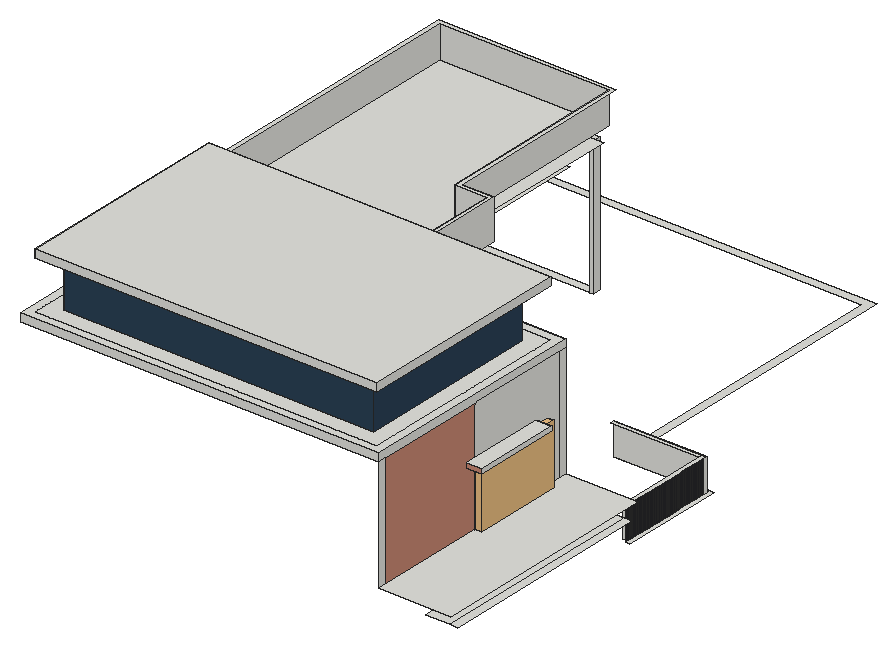
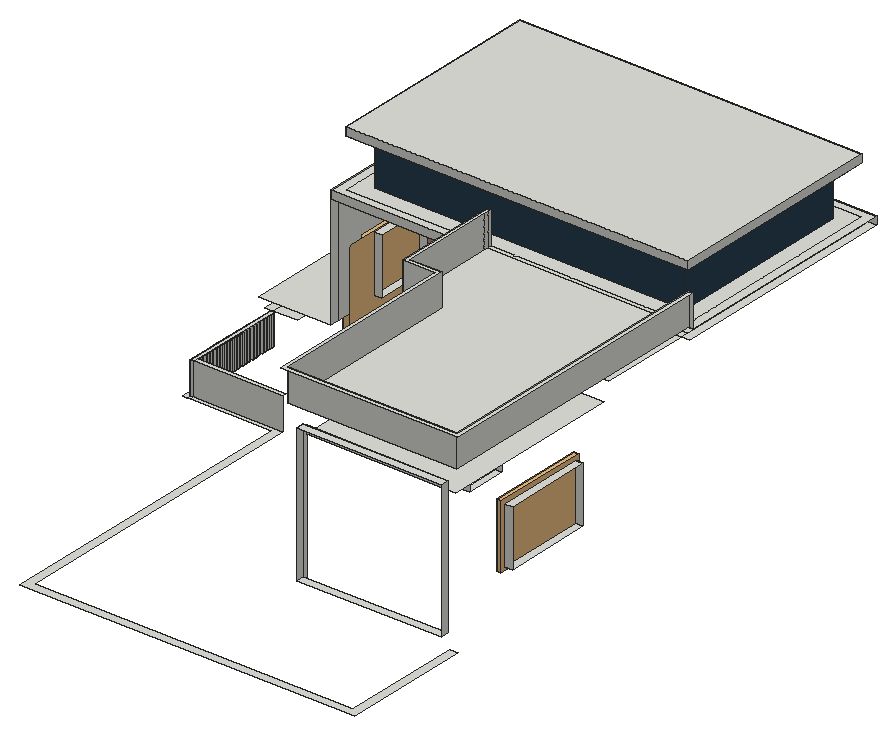
# SketchUp Ruby script. Lengths in inches.
U = 1.inch
M = Sketchup.active_model
def pt(a) = Geom::Point3d.new(a.map { |v| v * U })
def face(e, loops, mat)
  f = e.add_face(loops[0].map { |a| pt(a) })
  loops[1..].each { |l| e.add_face(l.map { |a| pt(a) }).erase! }
  f.material = f.back_material = mat if mat
  f
end
# faces: each face lists its corners as indices into pts; further lists are holes
def faces(e, pts, list, mat = nil) = list.each { |f| face(e, (f[0].is_a?(Array) ? f : [f]).map { |l| l.map { |i| pts[i] } }, mat) }
# xy, xz, yz: faces in a plane at the given z, y or x. An outline is a flat list of corners, or four numbers for a rectangle; further outlines are holes
def ring(l) = l.size == 4 ? [[l[0], l[1]], [l[2], l[1]], [l[2], l[3]], [l[0], l[3]]] : l.each_slice(2).to_a
def flat(e, list, mat, &to3) = list.each { |f| face(e, (f[0].is_a?(Array) ? f : [f]).map { |l| ring(l).map { |u, v| to3.(u, v) } }, mat) }
def xy(e, z, list, mat = nil) = flat(e, list, mat) { |x, y| [x, y, z] }
def xz(e, y, list, mat = nil) = flat(e, list, mat) { |x, z| [x, y, z] }
def yz(e, x, list, mat = nil) = flat(e, list, mat) { |y, z| [x, y, z] }
def lines(e, pts, list) = list.each { |a, b| e.add_line(pt(pts[a]), pt(pts[b])) }
# prism: a flat outline (further loops are holes) pulled along v
def prism(e, loops, v, mat = nil)
  f = face(e, loops, mat); d = Geom::Vector3d.new(v.map { |x| x * U })
  f.pushpull(f.normal.samedirection?(d) ? d.length : -d.length)
end
def box(e, o, s, mat = nil) = prism(e, [[o, [o[0] + s[0], o[1], o[2]], [o[0] + s[0], o[1] + s[1], o[2]], [o[0], o[1] + s[1], o[2]]]], [0, 0, s[2]], mat)
def at(x, y, z, deg = 0) = Geom::Transformation.translation(pt([x, y, z])) * Geom::Transformation.rotation(ORIGIN, Z_AXIS, deg.degrees)
def axes(o, x, y, z) = Geom::Transformation.new([*x, 0, *y, 0, *z, 0, *pt(o).to_a, 1])
def part(name) = M.definitions.add(name)
# library, detail: a bought-in or finely detailed component or shape, given as its bounding box
def library(name, o, s) = part(name).tap { |d| box(d.entities, o, s) }
def detail(e, o, s) = box(e.add_group.entities, o, s)
def put(e, d, t, mat = nil) = e.add_instance(d, t).tap { |i| i.material = mat if mat }
def group(e, t, mat = nil) = e.add_group.tap { |g| g.transformation = t; g.material = mat if mat }.entities
root = M.entities
M.materials.add("Brick_10_1K").color = [200, 136, 115]
M.materials.add("Carpet_04_1K").color = [43, 65, 85]
M.materials.add("ThomThom - Buttons2").color = [40, 40, 43]
c1 = library("mesh-162",[-1607.75,-1245.64,-53.98],[1739.16,1702.88,120.91])
c2 = part("Group9\#1")
put(c2.entities,c1,at(0,0,0))
xy(root,129,[[162,247.5,166.5,277.5]])
xy(root,132,[[357,219,360,297],[288,294,354,294,354,297,294,297,294,531,45,531,45,435,51,435,51,525,288,525],[354,294,357,297]])
xy(root,133,[[354,220,357,221.125],[354,223.125,357,224.25],[354,226.25,357,227.375],[354,229.375,357,230.5],[354,232.5,357,233.625],
  [354,235.625,357,236.75],[354,238.75,357,239.875],[354,241.875,357,243],[354,245,357,246.125],[354,248.125,357,249.25],
  [354,251.25,357,252.375],[354,254.375,357,255.5],[354,257.5,357,258.625],[354,260.625,357,261.75],[354,263.75,357,264.875],
  [354,266.875,357,268],[354,270,357,271.125],[354,273.125,357,274.25],[354,276.25,357,277.375],[354,279.375,357,280.5],
  [354,282.5,357,283.625],[354,285.625,357,286.75],[354,288.75,357,289.875]])
xy(root,138,[[57,429,165,435]])
xy(root,151.99,[[342,51,360,213],[360,51,366,213]])
xy(root,155,[[354,220,357,221.125],[354,223.125,357,224.25],[354,226.25,357,227.375],[354,229.375,357,230.5],[354,232.5,357,233.625],
  [354,235.625,357,236.75],[354,238.75,357,239.875],[354,241.875,357,243],[354,245,357,246.125],[354,248.125,357,249.25],
  [354,251.25,357,252.375],[354,254.375,357,255.5],[354,257.5,357,258.625],[354,260.625,357,261.75],[354,263.75,357,264.875],
  [354,266.875,357,268],[354,270,357,271.125],[354,273.125,357,274.25],[354,276.25,357,277.375],[354,279.375,357,280.5],
  [354,282.5,357,283.625],[354,285.625,357,286.75],[354,288.75,357,289.875]])
xy(root,156,[[354,219,357,294],[288,291,354,294]])
xy(root,162,[[312,45,366,219]])
xy(root,165,[[306,137.73,312,179.73],[45,318,51,384]])
xy(root,207,[[312,134.73,324,137.73],[306,137.73,324,179.73],[312,179.73,324,182.73],[312,182.73,324,191.34],[162,247.5,166.5,277.5],
  [45,318,51,384]])
xy(root,207,[[312,125.73,324,134.73]],"Brick_10_1K")
xy(root,210,[[312,125.73,324,191.34]])
xy(root,234,[[51,291,162,429],[162,291,166.5,405]])
xy(root,240,[[57,429,165,435]])
xy(root,246,[[45,45,51,219],[51,45,312,51],[51,51,178.5,213],[178.5,51,184.5,213],[184.5,51,306,213],
  [306,51,312,213],[51,213,312,219],[51,219,162,286.5],[166.5,219,201,286.5],[171,286.5,201,291],
  [166.5,291,177,423]])
xy(root,252,[[45,45,312,45,312,219,201,219,201,213,306,213,306,51,51,51,51,213,198,213,198,216,45,216],[[51,51,306,213],[63,63,294,201]],[69,69,288,195],[48,216,198,216,198,288,174,288,174,432,48,432]])
xy(root,276,[[198,213,201,213,201,291,177,291,177,435,45,435,45,216,48,216,48,432,174,432,174,288,198,288]])
xy(root,288,[[51,51,63,69],[63,51,306,63],[63,63,294,69],[294,63,306,69],[51,69,63,213],
  [63,69,69,201],[69,69,288,195],[288,69,294,201],[294,69,306,201],[69,195,288,201],
  [63,201,69,213],[69,201,288,213],[288,201,306,213]])
xy(root,294,[[51,51,306,213]])
xz(root,45,[[45,246,312,252]])
xz(root,51,[[51,288,306,294]])
xz(root,63,[[63,252,294,288]],"Carpet_04_1K")
xz(root,69,[[69,252,288,288]])
xz(root,125.73,[[312,207,324,210]],"Brick_10_1K")
xz(root,137.73,[[306,165,312,207]])
xz(root,179.73,[[306,165,312,207]])
xz(root,191.34,[[312,207,324,210]])
xz(root,195,[[69,252,288,288]])
xz(root,201,[[63,252,294,288]],"Carpet_04_1K")
xz(root,213,[[198,252,201,276],[51,288,306,294]])
xz(root,216,[[45,252,48,276]])
xz(root,219,[[201,246,312,252]])
xz(root,220,[[354,133,357,155]])
xz(root,221.125,[[354,133,357,155]])
xz(root,223.125,[[354,133,357,155]])
xz(root,224.25,[[354,133,357,155]])
xz(root,226.25,[[354,133,357,155]])
xz(root,227.375,[[354,133,357,155]])
xz(root,229.375,[[354,133,357,155]])
xz(root,230.5,[[354,133,357,155]])
xz(root,232.5,[[354,133,357,155]])
xz(root,233.625,[[354,133,357,155]])
xz(root,235.625,[[354,133,357,155]])
xz(root,236.75,[[354,133,357,155]])
xz(root,238.75,[[354,133,357,155]])
xz(root,239.875,[[354,133,357,155]])
xz(root,241.875,[[354,133,357,155]])
xz(root,243,[[354,133,357,155]])
xz(root,245,[[354,133,357,155]])
xz(root,246.125,[[354,133,357,155]])
xz(root,247.5,[[162,129,166.5,207]])
xz(root,248.125,[[354,133,357,155]])
xz(root,249.25,[[354,133,357,155]])
xz(root,251.25,[[354,133,357,155]])
xz(root,252.375,[[354,133,357,155]])
xz(root,254.375,[[354,133,357,155]])
xz(root,255.5,[[354,133,357,155]])
xz(root,257.5,[[354,133,357,155]])
xz(root,258.625,[[354,133,357,155]])
xz(root,260.625,[[354,133,357,155]])
xz(root,261.75,[[354,133,357,155]])
xz(root,263.75,[[354,133,357,155]])
xz(root,264.875,[[354,133,357,155]])
xz(root,266.875,[[354,133,357,155]])
xz(root,268,[[354,133,357,155]])
xz(root,270,[[354,133,357,155]])
xz(root,271.125,[[354,133,357,155]])
xz(root,273.125,[[354,133,357,155]])
xz(root,274.25,[[354,133,357,155]])
xz(root,276.25,[[354,133,357,155]])
xz(root,277.375,[[354,133,357,155]])
xz(root,277.5,[[162,129,166.5,207]])
xz(root,279.375,[[354,133,357,155]])
xz(root,280.5,[[354,133,357,155]])
xz(root,282.5,[[354,133,357,155]])
xz(root,283.625,[[354,133,357,155]])
xz(root,285.625,[[354,133,357,155]])
xz(root,286.75,[[354,133,357,155]])
xz(root,288,[[174,252,198,276]])
xz(root,288.75,[[354,133,357,155]])
xz(root,289.875,[[354,133,357,155]])
xz(root,291,[[177,246,201,276]])
xz(root,294,[[288,132,354,156],[354,132,357,156]])
xz(root,318,[[45,165,51,207]])
xz(root,384,[[45,165,51,207]])
xz(root,429,[[162,138,165,240],[57,234,162,240]])
xz(root,432,[[48,252,174,276]])
yz(root,48,[[216,252,432,276]])
yz(root,51,[[[315,162,387,210],[318,165,384,207]],[51,288,213,294]])
yz(root,57,[[429,138,435,240]])
yz(root,63,[[63,252,201,288]],"Carpet_04_1K")
yz(root,69,[[69,252,195,288]])
yz(root,165,[[429,138,435,240]])
yz(root,166.5,[[219,234,286.5,246]])
yz(root,174,[[288,252,432,276]])
yz(root,198,[[213,252,216,276],[216,252,219,276],[219,252,288,276]])
yz(root,201,[[219,246,291,276],[213,252,219,276]])
yz(root,288,[[69,252,195,288]])
yz(root,294,[[63,252,201,288]],"Carpet_04_1K")
yz(root,306,[[51,288,213,294]])
yz(root,312,[[45,162,51,246],[134.73,162,182.73,162,182.73,207,179.73,207,179.73,165,137.73,165,137.73,207,134.73,207],[182.73,162,213,162,213,246,134.73,246,134.73,210,191.34,210,191.34,207,182.73,207],[213,162,219,246],[45,246,219,252]])
yz(root,312,[[51,162,134.73,162,134.73,207,125.73,207,125.73,210,134.73,210,134.73,246,51,246]],"Brick_10_1K")
yz(root,324,[[125.73,207,191.34,210]])
yz(root,357,[[290.875,132,294,156]])
yz(root,357,[[[219,132,222.125,156],[220,133,221.125,155]],[[222.125,132,225.25,156],[223.125,133,224.25,155]],[[225.25,132,228.375,156],[226.25,133,227.375,155]],[[228.375,132,231.5,156],[229.375,133,230.5,155]],[[231.5,132,234.625,156],[232.5,133,233.625,155]],
  [[234.625,132,237.75,156],[235.625,133,236.75,155]],[[237.75,132,240.875,156],[238.75,133,239.875,155]],[[240.875,132,244,156],[241.875,133,243,155]],[[244,132,247.125,156],[245,133,246.125,155]],[[247.125,132,250.25,156],[248.125,133,249.25,155]],
  [[250.25,132,253.375,156],[251.25,133,252.375,155]],[[253.375,132,256.5,156],[254.375,133,255.5,155]],[[256.5,132,259.625,156],[257.5,133,258.625,155]],[[259.625,132,262.75,156],[260.625,133,261.75,155]],[[262.75,132,265.875,156],[263.75,133,264.875,155]],
  [[265.875,132,269,156],[266.875,133,268,155]],[[269,132,272.125,156],[270,133,271.125,155]],[[272.125,132,275.25,156],[273.125,133,274.25,155]],[[275.25,132,278.375,156],[276.25,133,277.375,155]],[[278.375,132,281.5,156],[279.375,133,280.5,155]],
  [[281.5,132,284.625,156],[282.5,133,283.625,155]],[[284.625,132,287.75,156],[285.625,133,286.75,155]],[[287.75,132,290.875,156],[288.75,133,289.875,155]]],"ThomThom - Buttons2")
p = [[166.5,291,234],[166.5,286.5,234]]
lines(root,p,[[0,1]])
g1 = group(root,at(314.63,183.77,201.83))
put(g1,c1,axes([0,0,0],[0,0,0.03937],[0,0.03937,0],[-0.03937,0,0]))
put(root,c2,axes([52.84,367.67,206.38],[0,0,0.02756],[0,0.04228,0],[-0.02756,0,0]))
